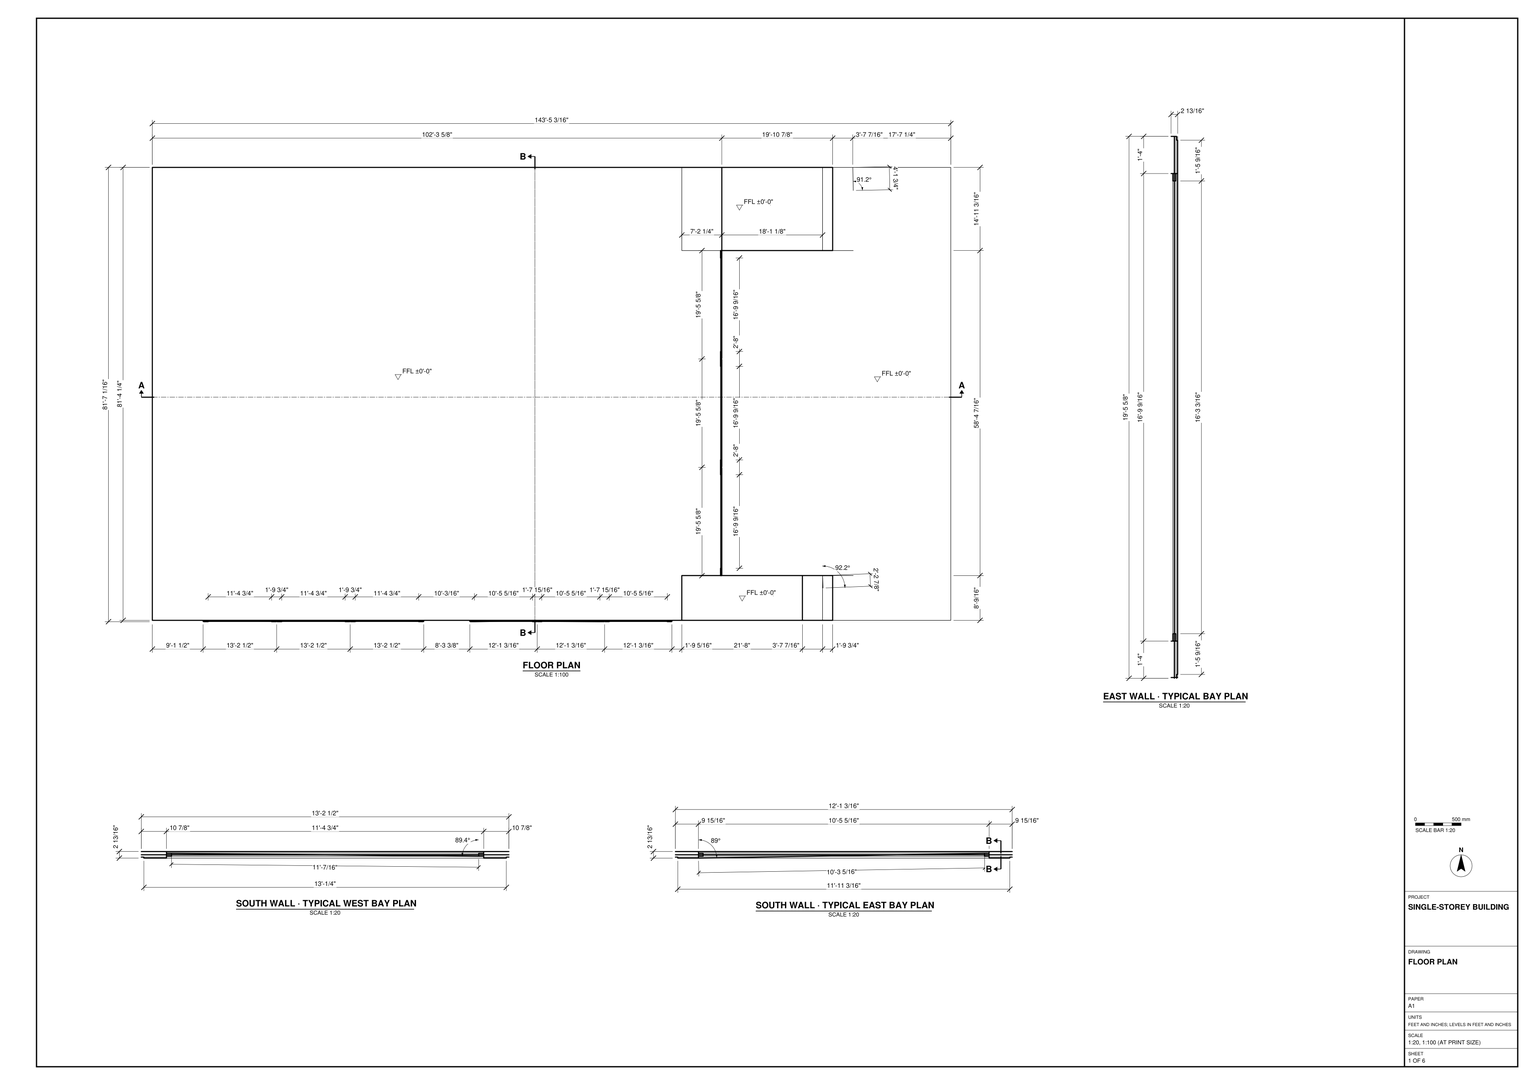
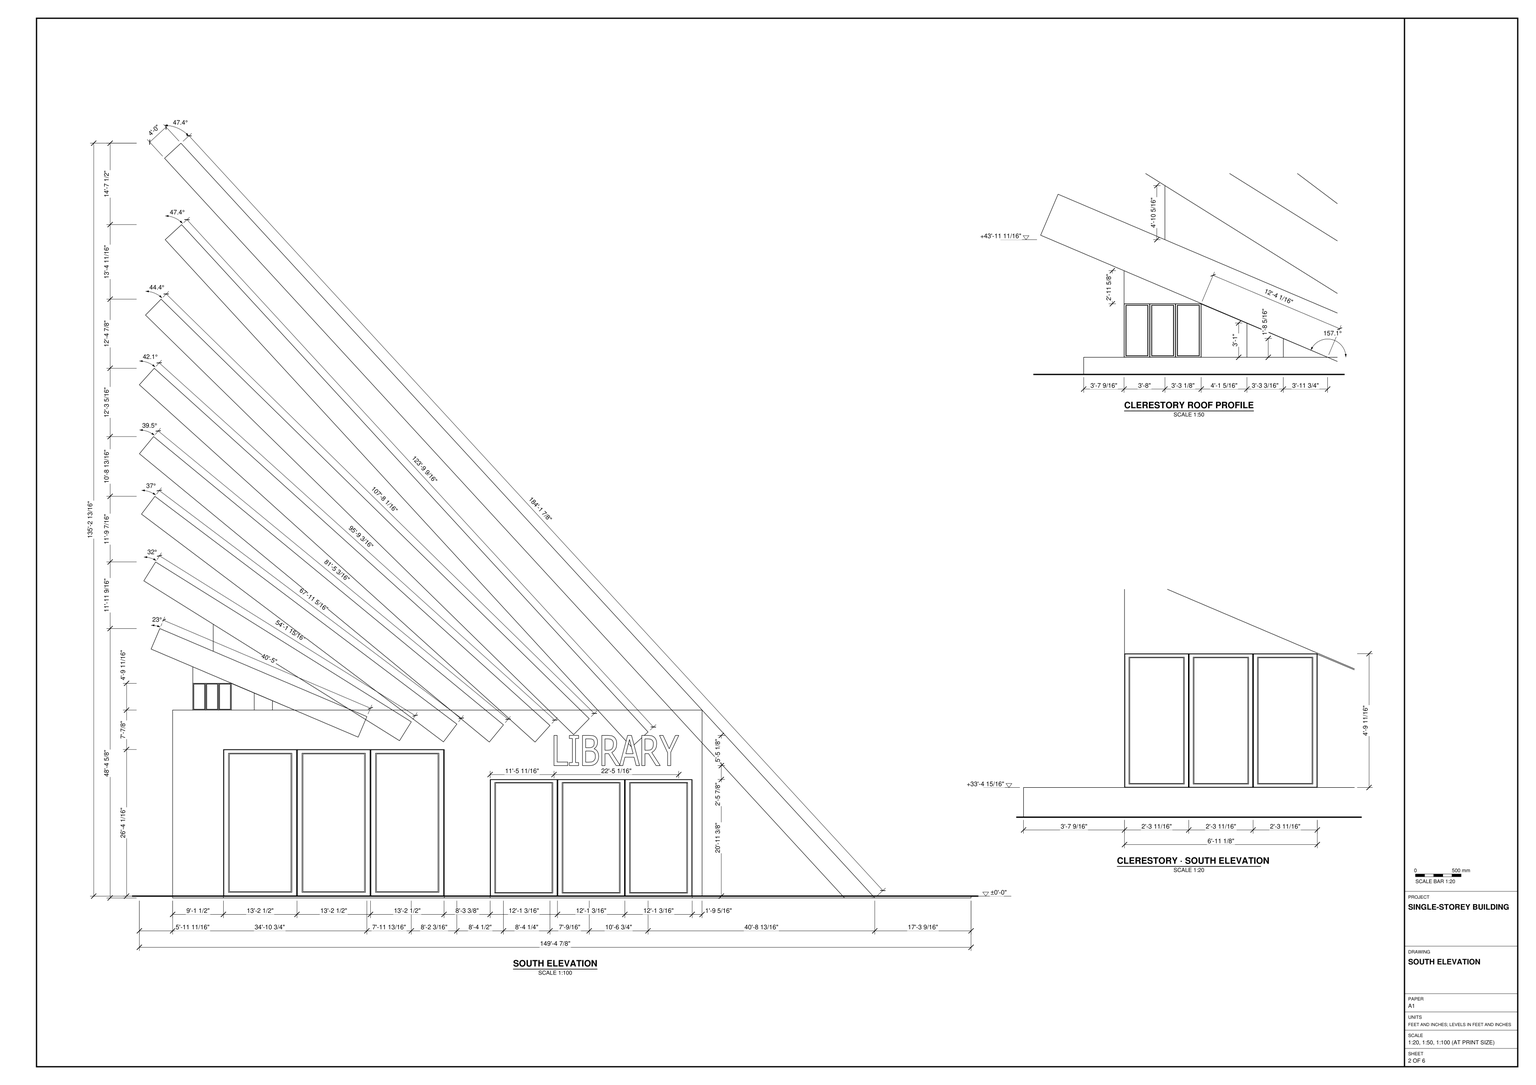
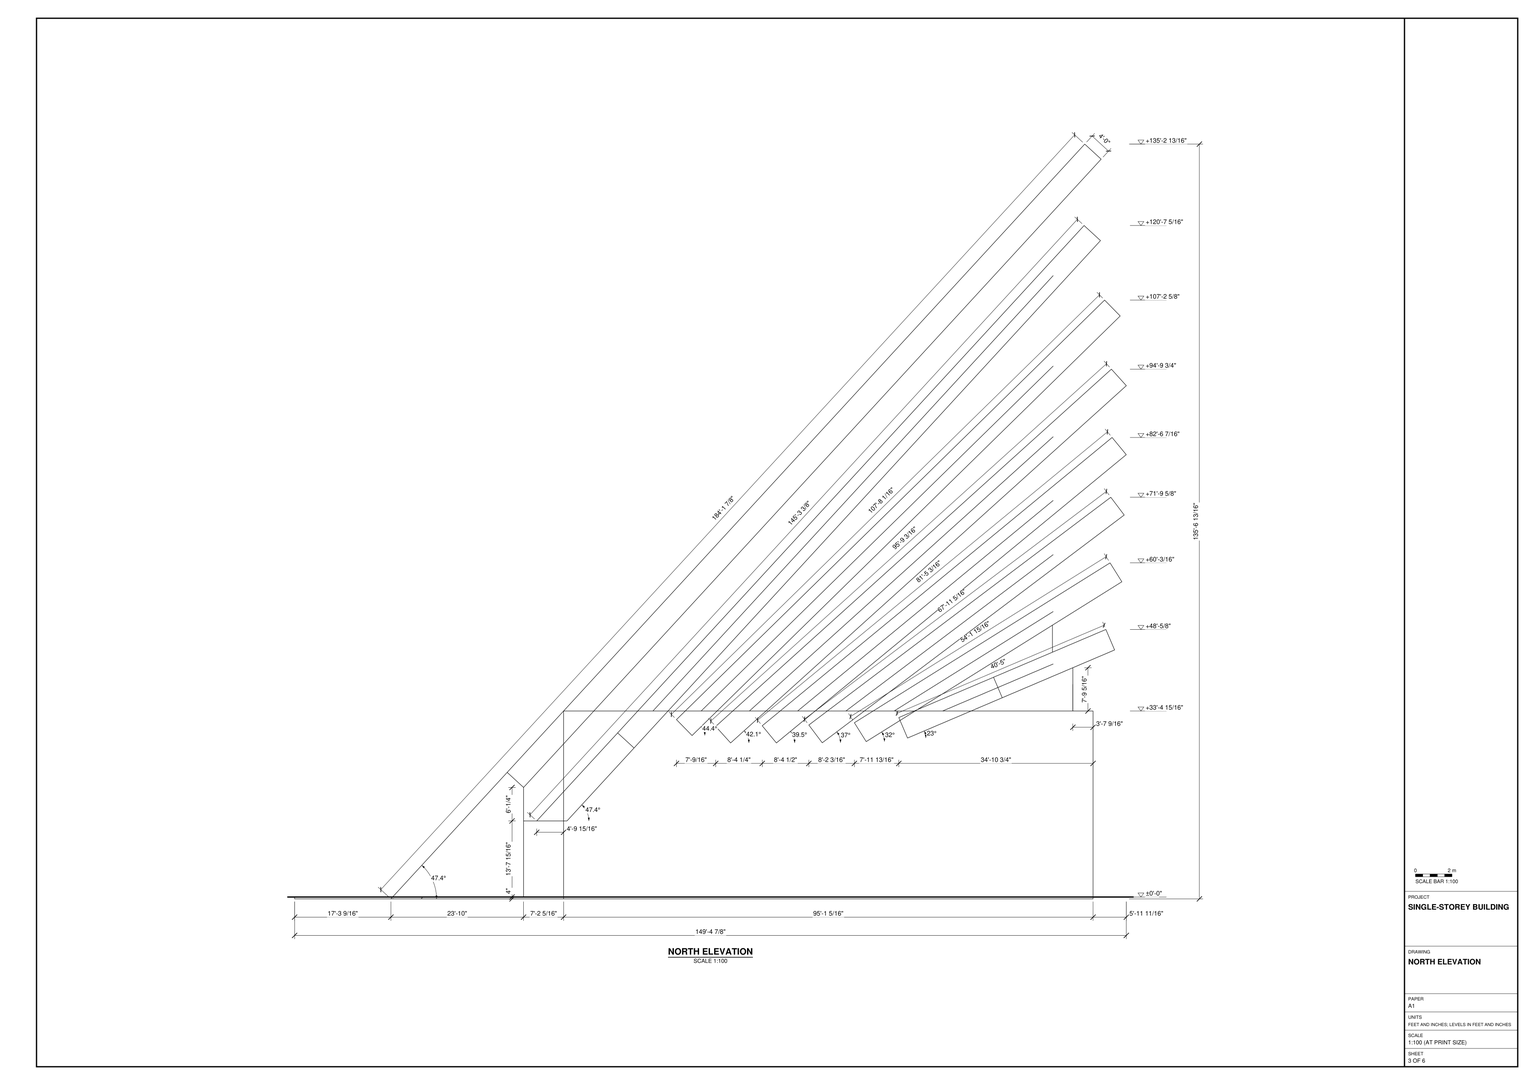
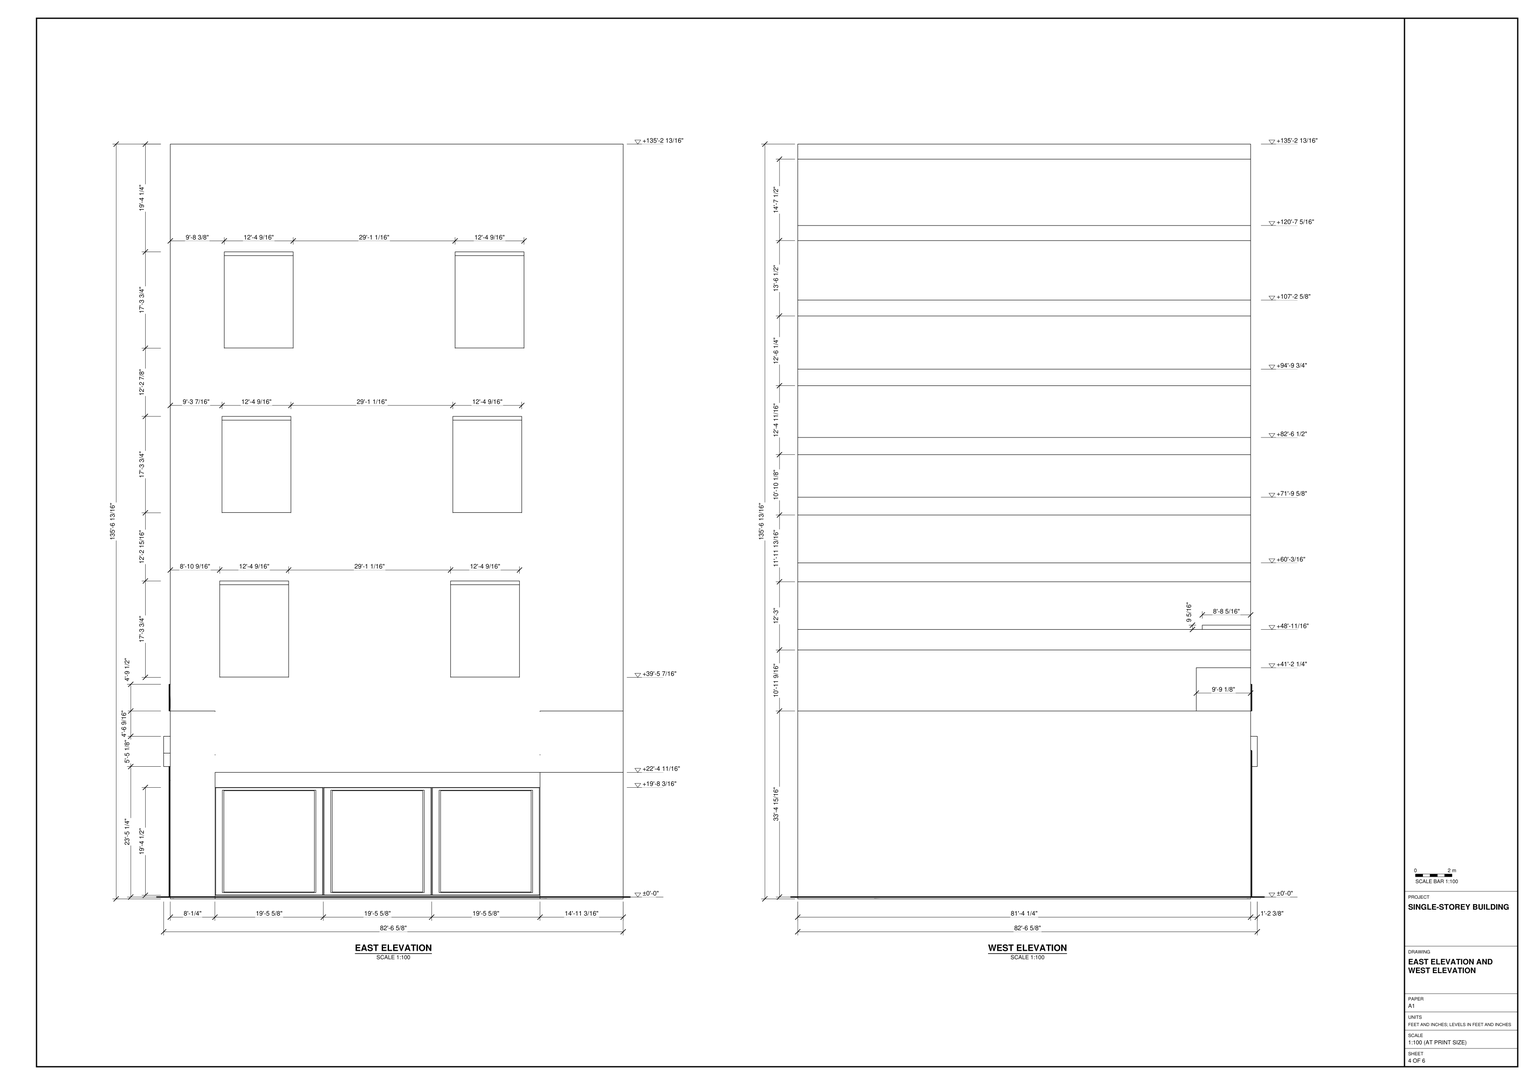
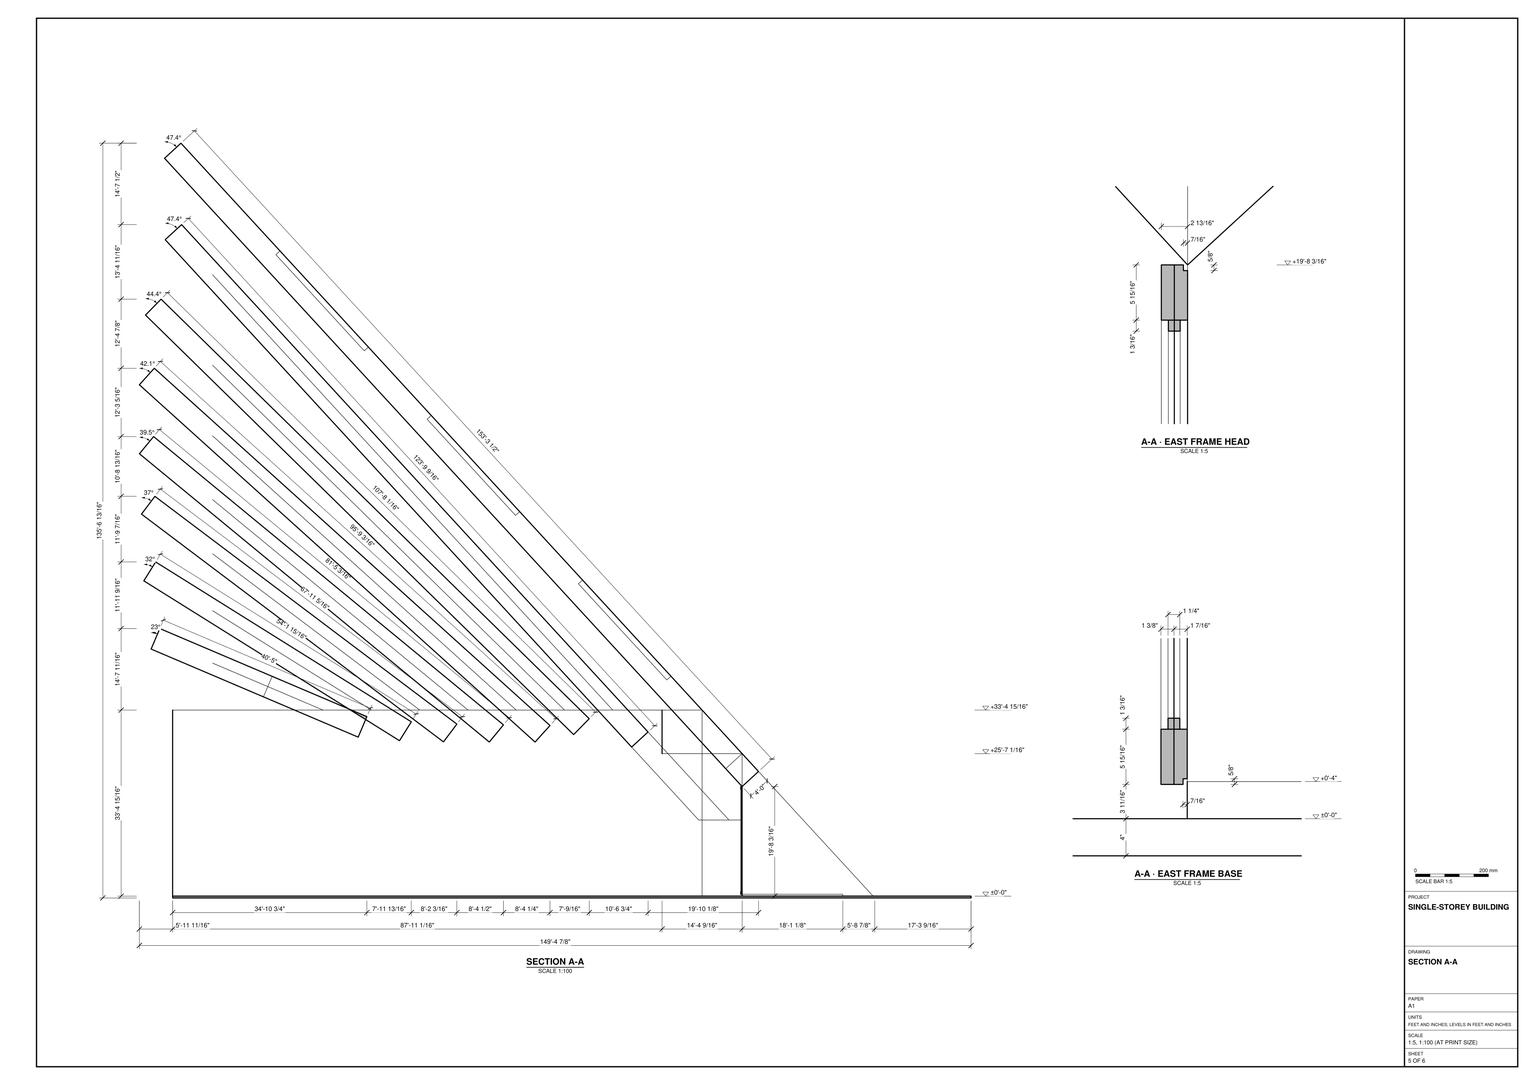
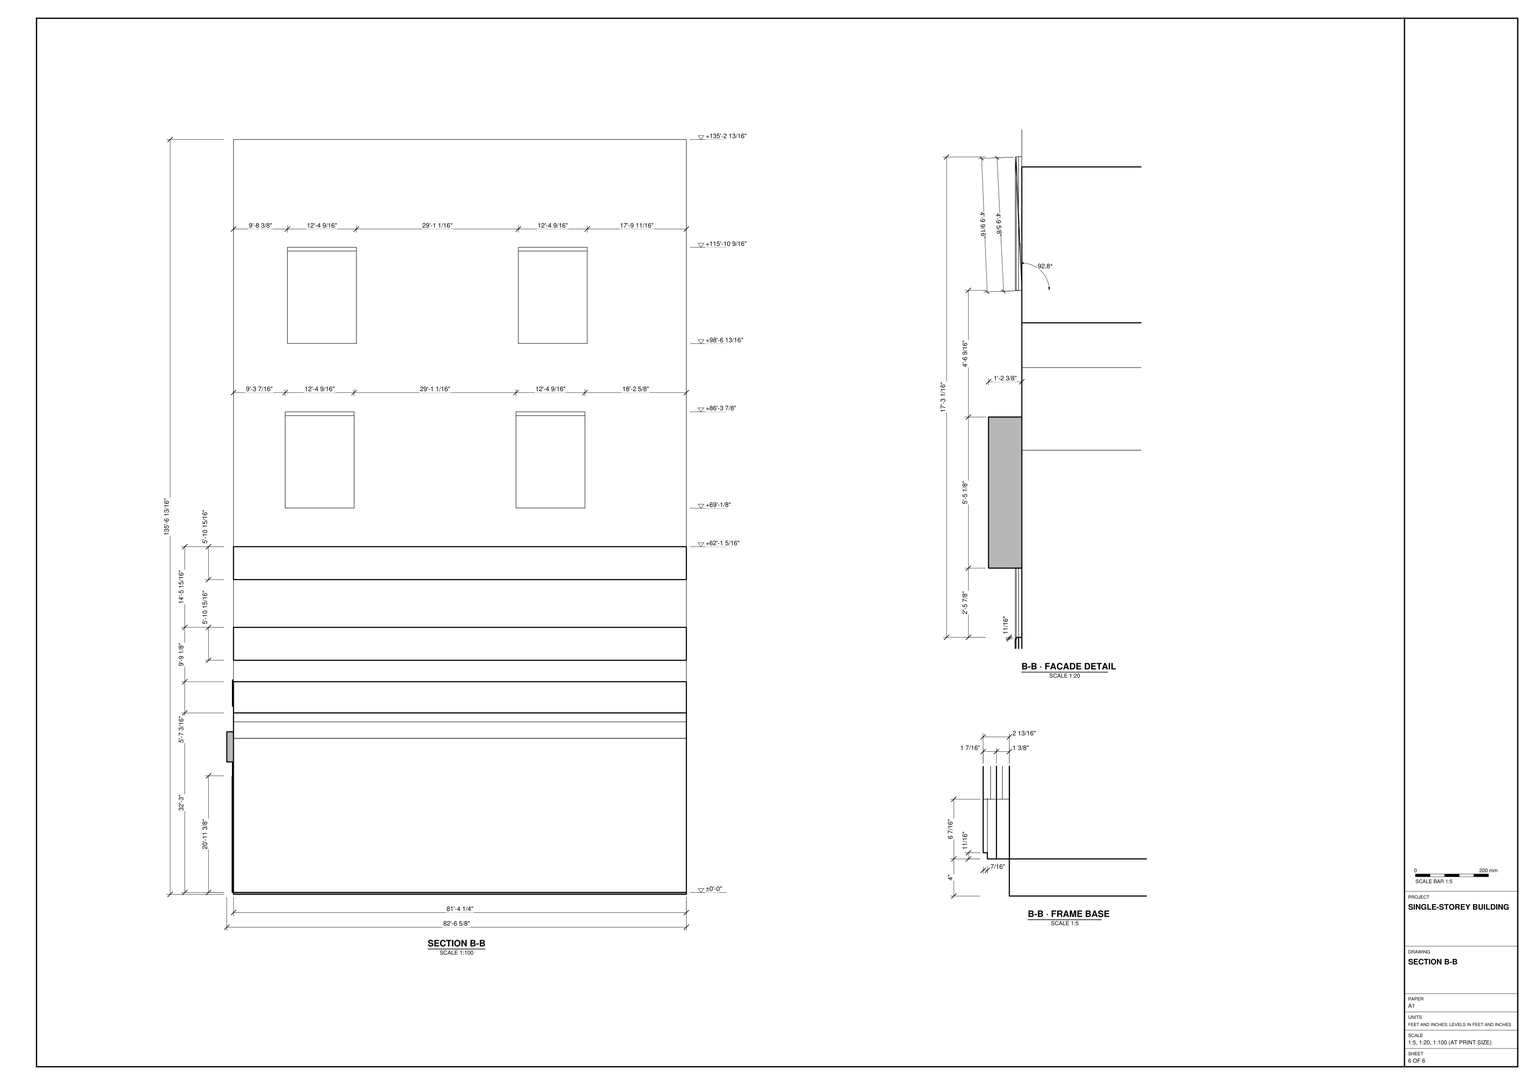
Build the single-storey library in SketchUp from task_files/diagram_01.pdf. Work in feet and inches. The overall model extents are 149'-4 7/8" east to west, 82'-6 5/8" north to south and 135'-6 13/16" vertically. Set the finished ground floor at ±0'-0".

Lay out the slab and walls from the floor plan, including the recessed east wall between the projecting ends. Use the typical bay plans to set the wall and frame thicknesses. On the south wall, form the taller bank of glazed bays to the west and the lower bank to the east, with the library lettering above the lower bank. Keep the broad north wall plain as shown in elevation.

Use the north and south elevations together to set out the inclined roof elements. Give each its drawn thickness, slope and endpoints so that the separate tips form a fan above the building and the longest element reaches the slab to the east. Fit the framed clerestory glazing beneath the lowest inclined element.

Keep walls, slabs, roof elements and any furniture or joinery pieces in separate groups or components, and use components for repeated parts. Decor and loose items may be suitable library components. Save one SketchUp model as output_files/single_storey_library_with_a_fan_shaped_roof.skp.

# SketchUp Ruby script. Lengths in inches.
U = 1.inch
M = Sketchup.active_model
def pt(a) = Geom::Point3d.new(a.map { |v| v * U })
def face(e, loops, mat)
  f = e.add_face(loops[0].map { |a| pt(a) })
  loops[1..].each { |l| e.add_face(l.map { |a| pt(a) }).erase! }
  f.material = f.back_material = mat if mat
  f
end
# faces: each face lists its corners as indices into pts; further lists are holes
def faces(e, pts, list, mat = nil) = list.each { |f| face(e, (f[0].is_a?(Array) ? f : [f]).map { |l| l.map { |i| pts[i] } }, mat) }
# xy, xz, yz: faces in a plane at the given z, y or x. An outline is a flat list of corners, or four numbers for a rectangle; further outlines are holes
def ring(l) = l.size == 4 ? [[l[0], l[1]], [l[2], l[1]], [l[2], l[3]], [l[0], l[3]]] : l.each_slice(2).to_a
def flat(e, list, mat, &to3) = list.each { |f| face(e, (f[0].is_a?(Array) ? f : [f]).map { |l| ring(l).map { |u, v| to3.(u, v) } }, mat) }
def xy(e, z, list, mat = nil) = flat(e, list, mat) { |x, y| [x, y, z] }
def xz(e, y, list, mat = nil) = flat(e, list, mat) { |x, z| [x, y, z] }
def yz(e, x, list, mat = nil) = flat(e, list, mat) { |y, z| [x, y, z] }
def lines(e, pts, list) = list.each { |a, b| e.add_line(pt(pts[a]), pt(pts[b])) }
# prism: a flat outline (further loops are holes) pulled along v
def prism(e, loops, v, mat = nil)
  f = face(e, loops, mat); d = Geom::Vector3d.new(v.map { |x| x * U })
  f.pushpull(f.normal.samedirection?(d) ? d.length : -d.length)
end
def box(e, o, s, mat = nil) = prism(e, [[o, [o[0] + s[0], o[1], o[2]], [o[0] + s[0], o[1] + s[1], o[2]], [o[0], o[1] + s[1], o[2]]]], [0, 0, s[2]], mat)
def at(x, y, z, deg = 0) = Geom::Transformation.translation(pt([x, y, z])) * Geom::Transformation.rotation(ORIGIN, Z_AXIS, deg.degrees)
def axes(o, x, y, z) = Geom::Transformation.new([*x, 0, *y, 0, *z, 0, *pt(o).to_a, 1])
def part(name) = M.definitions.add(name)
# library, detail: a bought-in or finely detailed component or shape, given as its bounding box
def library(name, o, s) = part(name).tap { |d| box(d.entities, o, s) }
def detail(e, o, s) = box(e.add_group.entities, o, s)
def put(e, d, t, mat = nil) = e.add_instance(d, t).tap { |i| i.material = mat if mat }
def group(e, t, mat = nil) = e.add_group.tap { |g| g.transformation = t; g.material = mat if mat }.entities
root = M.entities
M.materials.add("Wine2").color = [0, 0, 0]
M.materials["Wine2"].alpha = 0
M.materials.add("[0130_Gainsboro]").color = [39, 45, 50]
M.materials.add("[Slate]").color = [102, 110, 108]
M.materials.add("[Translucent Glass Safety]").color = [204, 235, 244]
M.materials["[Translucent Glass Safety]"].alpha = 0.5
c1 = part("Framed glazing panel")
xy(c1.entities,0,[[0,-0.98,43.07,0],[0,0,43.07,1.4]],"[0130_Gainsboro]")
xy(c1.entities,0.3,[[0.3,-1.43,42.77,-0.98]],"[0130_Gainsboro]")
xy(c1.entities,2.95,[[2.95,-1.43,40.12,-0.63],[2.95,-0.63,40.12,0],[2.95,0,40.12,0.64],[2.95,0.64,40.12,1.4]],"[0130_Gainsboro]")
xy(c1.entities,3.54,[[3.54,-0.63,39.53,0],[3.54,0,39.53,0.64]],"[0130_Gainsboro]")
xy(c1.entities,111.8125,[[3.54,-0.63,39.53,0],[3.54,0,39.53,0.64]],"[0130_Gainsboro]")
xy(c1.entities,112.4,[[2.95,-1.43,40.12,-0.63],[2.95,-0.63,40.12,0],[2.95,0,40.12,0.64],[2.95,0.64,40.12,1.4]],"[0130_Gainsboro]")
xy(c1.entities,115.05,[[0.3,-1.43,42.77,-0.98]],"[0130_Gainsboro]")
xy(c1.entities,115.35,[[0,-0.98,43.07,0],[0,0,43.07,1.4]],"[0130_Gainsboro]")
xz(c1.entities,-1.43,[[[0.3,0.3,42.77,115.05],[2.95,2.95,40.12,112.4]]],"[0130_Gainsboro]")
xz(c1.entities,-0.98,[[[0,0,43.07,115.35],[0.3,0.3,42.77,115.05]]],"[0130_Gainsboro]")
xz(c1.entities,-0.63,[[[2.95,2.95,40.12,112.4],[3.54,3.54,39.53,111.8125]]],"[0130_Gainsboro]")
xz(c1.entities,0,[[3.54,3.54,39.53,111.8125]],"Wine2")
xz(c1.entities,0,[[[0,0,43.07,115.35],[2.95,2.95,40.12,112.4]],[[2.95,2.95,40.12,112.4],[3.54,3.54,39.53,111.8125]]],"[0130_Gainsboro]")
xz(c1.entities,0.64,[[[2.95,2.95,40.12,112.4],[3.54,3.54,39.53,111.8125]]],"[0130_Gainsboro]")
xz(c1.entities,1.4,[[[0,0,43.07,115.35],[2.95,2.95,40.12,112.4]]],"[0130_Gainsboro]")
yz(c1.entities,0,[[-0.98,0,0,115.35],[0,0,1.4,115.35]],"[0130_Gainsboro]")
yz(c1.entities,0.3,[[-1.43,0.3,-0.98,115.05]],"[0130_Gainsboro]")
yz(c1.entities,2.95,[[-1.43,2.95,-0.63,112.4],[-0.63,2.95,0,112.4],[0,2.95,0.64,112.4],[0.64,2.95,1.4,112.4]],"[0130_Gainsboro]")
yz(c1.entities,3.54,[[-0.63,3.54,0,111.8125],[0,3.54,0.64,111.8125]],"[0130_Gainsboro]")
yz(c1.entities,39.53,[[-0.63,3.54,0,111.8125],[0,3.54,0.64,111.8125]],"[0130_Gainsboro]")
yz(c1.entities,40.12,[[-1.43,2.95,-0.63,112.4],[-0.63,2.95,0,112.4],[0,2.95,0.64,112.4],[0.64,2.95,1.4,112.4]],"[0130_Gainsboro]")
yz(c1.entities,42.77,[[-1.43,0.3,-0.98,115.05]],"[0130_Gainsboro]")
yz(c1.entities,43.07,[[-0.98,0,0,115.35],[0,0,1.4,115.35]],"[0130_Gainsboro]")
c2 = part("Glazed panel assembly")
put(c2.entities,c1,axes([90.57,1.43,0],[1.05148,0,0],[0,1,0],[0,0,1]))
put(c2.entities,c1,axes([0,1.43,0],[1.05148,0,0],[0,1,0],[0,0,1]))
put(c2.entities,c1,axes([45.29,1.43,0],[1.05148,0,0],[0,1,0],[0,0,1]))
c3 = library("LIBRARY",[0.96,0,0],[49.83,9.51,1])
prism(root,[[[936.12,2.83,184.17],[13.24,2.83,1088.42],[13.24,979.08,1088.42],[936.12,979.08,184.17]]],[33.59,0,34.29])
prism(root,[[[852.98,2.83,168.11],[0,2.83,938.18],[0,979.08,938.18],[852.98,979.08,168.11]]],[32.17,0,35.63])
prism(root,[[[754.34,2.83,168.13],[0.15,2.83,789.49],[0.15,979.08,789.49],[754.34,979.08,168.13]]],[30.52,0,37.05])
prism(root,[[[655.5,2.83,168.46],[4.59,2.83,659.39],[4.59,979.08,659.39],[655.5,979.08,168.46]]],[28.9,0,38.32])
xy(root,-167.93,[[71.7,2.83,1792.87,979.08]])
xy(root,-163.93,[[1213.03,2.83,1516.4375,99.4],[1516.4375,2.83,1792.87,2.83,1792.87,979.08,1516.4375,979.08,1516.4375,799.87,1299.3,799.87,1299.3,99.4,1516.4375,99.4],[1299.3,799.87,1516.4375,979.08]])
xy(root,237,[[115.23,2.83,334.62,119.96]])
xz(root,1.43,[[117.51,238.77,140.66,292.91],[145.22,238.77,168.37,292.91],[172.92,238.77,196.08,292.91]])
xz(root,2.83,[[71.7,-167.93,181.19,-163.93],[181.19,-167.93,657.38,152.13],[657.38,-167.93,756.09,-163.93],[756.09,-167.93,1191.71,87.44],[1191.71,-167.93,1520.11,-167.93,1516.4375,-163.93,1191.71,-163.93],
  [1520.11,-167.93,1585.32,-167.93,1581.64,-163.93,1516.4375,-163.93],[1585.32,-167.93,1792.87,-167.93,1792.87,-163.93,1581.64,-163.93],[1516.4375,-163.93,1581.64,-163.93,89.64,1458.875,54.31,1426.39,1213.03,166.08],[1213.03,-163.93,1516.4375,-163.93,1213.03,166.08],[1061.15,157.3125,1096.48,189.8,91.04,1283.4,55.7,1250.91],
  [560.76,171.01,586.21,211.72,35.08,556.26,9.63,515.56,159.23,422.03,450.84,239.73,490.42,222.9,487.76,216.65],[471.64,178.73,487.76,216.65,450.84,239.73,159.23,363.76,44.09,412.73,25.3,368.56,115.23,330.31,334.62,237],[487.76,216.65,490.42,222.9,450.84,239.73]])
xz(root,2.83,[[115.23,237,334.62,237,115.23,330.31],[450.84,239.73,159.23,422.03,159.23,363.76]],"[Translucent Glass Safety]")
xz(root,99.4,[[1585.32,-167.93,1516.4375,-163.93,1516.4375,-159.93,1512.76,-159.93,1299.3,72.24,1334.64,104.72],[1213.03,-163.93,1299.3,-159.93],[1299.3,-163.93,1299.3,-159.93,1512.76,-159.93,1516.4375,-163.93],[1516.4375,-163.93,1512.76,-159.93,1516.4375,-159.93],[1213.03,-159.93,1213.03,143.16,1299.3,143.16,1263.97,110.67,1299.3,72.24,1512.76,-159.93],
  [1299.3,72.24,1263.97,110.67,1299.3,143.16]])
xz(root,107.14,[[450.84,239.73,159.23,422.03,159.23,363.76]])
xz(root,109.39,[[1136.98,301.99,946.5,509.17,955.33,517.29,1145.8125,310.11]])
xz(root,114.29,[[810.9,656.66,620.42,863.84,629.25,871.96,819.73,664.78]])
xz(root,119.18,[[484.82,1011.32,294.33,1218.51,303.17,1226.63,493.65,1019.45]])
xz(root,119.96,[[115.23,237,115.23,330.31,334.62,237]])
xz(root,257.95,[[1136.98,301.99,1145.8125,310.11,955.33,517.29,946.5,509.17]])
xz(root,262.85,[[810.9,656.66,819.73,664.78,629.25,871.96,620.42,863.84]])
xz(root,267.75,[[484.82,1011.32,493.65,1019.45,303.17,1226.63,294.33,1218.51]])
xz(root,607.01,[[1136.98,301.99,946.5,509.17,955.33,517.29,1145.8125,310.11]])
xz(root,611.91,[[810.9,656.66,620.42,863.84,629.25,871.96,819.73,664.78]])
xz(root,616.81,[[484.82,1011.32,294.33,1218.51,303.17,1226.63,493.65,1019.45]])
xz(root,755.58,[[1136.98,301.99,1145.8125,310.11,955.33,517.29,946.5,509.17]])
xz(root,760.47,[[810.9,656.66,819.73,664.78,629.25,871.96,620.42,863.84]])
xz(root,765.37,[[484.82,1011.32,493.65,1019.45,303.17,1226.63,294.33,1218.51]])
xz(root,799.87,[[1520.11,-167.93,1585.32,-167.93,1334.64,104.72,1299.3,72.24,1299.3,-159.93,1516.4375,-159.93,1516.4375,-163.93],[1299.3,-163.93,1516.4375,-159.93],[1299.3,72.24,1299.3,143.16,1263.97,110.67]])
xz(root,979.08,[[71.7,-167.93,1213.03,-163.93],[1213.03,-167.93,1213.03,0,1299.3,0,1299.3,-163.93,1516.4375,-163.93,1520.11,-167.93],[1520.11,-167.93,1516.4375,-163.93,1581.64,-163.93,1585.32,-167.93],[1585.32,-167.93,1581.64,-163.93,1792.87,-163.93,1792.87,-167.93],[1299.3,-163.93,1299.3,72.24,1334.64,104.72,1581.64,-163.93],
  [1205.78,0,1061.15,157.3125,1096.48,189.8,1213.03,63.04,1213.03,0],[1213.03,0,1213.03,63.04,1270.98,0],[1270.98,0,1213.03,63.04,1213.03,166.08,1299.3,72.24,1299.3,0],[1299.3,72.24,1334.64,104.72,89.64,1458.875,54.31,1426.39,1213.03,166.08],[1061.15,157.3125,55.7,1250.91,91.04,1283.4,1096.48,189.8],
  [560.76,171.01,487.76,216.65,490.42,222.9,450.84,239.73,9.63,515.56,35.08,556.26,586.21,211.72],[471.64,178.73,267.46,265.57,286.25,309.74,450.84,239.73,487.76,216.65],[487.76,216.65,450.84,239.73,490.42,222.9],[267.46,265.57,25.3,368.56,44.09,412.73,286.25,309.74]])
yz(root,71.7,[[2.83,-167.93,979.08,-163.93]])
yz(root,115.23,[[2.83,237,119.96,330.31]])
yz(root,159.23,[[2.83,363.76,107.14,422.03]])
yz(root,1126.75,[[99.4,143.16,799.87,237]])
yz(root,1213.03,[[2.83,-163.93,99.4,166.08]])
yz(root,1299.3,[[99.4,-163.93,799.87,-159.93],[799.87,-163.93,979.08,0],[799.87,0,979.08,72.24]])
yz(root,1299.3,[[115.1,-154.29,316.66,66.29],[348.69,-154.29,550.26,66.29],[582.29,-154.29,783.85,66.29]],"[Translucent Glass Safety]")
yz(root,1792.87,[[2.83,-167.93,99.4,-163.93],[99.4,-167.93,799.87,-163.93],[799.87,-167.93,979.08,-163.93]])
p = [[1581.64,2.83,-163.93],[1585.32,2.83,-167.93],[1585.32,99.4,-167.93],[1334.64,99.4,104.72],[1334.64,799.87,104.72],[1334.64,979.08,104.72],
  [89.64,979.08,1458.875],[89.64,2.83,1458.875],[955.33,257.95,517.29],[1145.8125,257.95,310.11],[1145.8125,109.39,310.11],[955.33,109.39,517.29],
  [303.17,765.37,1226.63],[493.65,765.37,1019.45],[493.65,616.81,1019.45],[303.17,616.81,1226.63],[629.25,760.47,871.96],[819.73,760.47,664.78],
  [819.73,611.91,664.78],[629.25,611.91,871.96],[629.25,262.85,871.96],[819.73,262.85,664.78],[819.73,114.29,664.78],[629.25,114.29,871.96],
  [955.33,755.58,517.29],[1145.8125,755.58,310.11],[1145.8125,607.01,310.11],[955.33,607.01,517.29],[303.17,119.18,1226.63],[303.17,267.75,1226.63],
  [493.65,267.75,1019.45],[493.65,119.18,1019.45],[1516.4375,2.83,-163.93],[1516.4375,99.4,-163.93],[1520.11,2.83,-167.93],[1585.32,799.87,-167.93],
  [1581.64,979.08,-163.93],[1299.3,979.08,72.24],[1299.3,799.87,72.24],[1263.97,799.87,110.67],[1263.97,99.4,110.67],[1299.3,99.4,72.24],
  [1512.76,99.4,-159.93],[1213.03,2.83,166.08],[54.31,2.83,1426.39],[54.31,979.08,1426.39],[1213.03,979.08,166.08],[911.25,0.8125,-157.5],
  [911.25,0.8125,81.01],[1036.55,0.01,81.01],[1036.55,0.01,-157.5],[1058.44,2.08,-157.5],[1058.44,2.08,79.73],[1181.76,1.44,79.73],
  [1181.76,1.44,-157.5],[766.04,0.01,-156.22],[766.04,0.01,81.01],[889.36,2.08,81.01],[889.36,2.08,-156.22],[326.67,0.8,-154.23],
  [194.22,2.07,-154.23],[194.22,2.07,142.43],[326.67,0.8,142.43],[352.73,2.07,142.43],[485.17,0.8,142.43],[485.17,0.8,-154.23],
  [352.73,2.07,-154.23],[511.23,2.07,-154.23],[511.23,2.07,142.43],[643.68,0.8,142.43],[643.68,0.8,-154.23],[55.7,979.08,1250.91],
  [1061.15,979.08,157.3125],[1061.15,2.83,157.3125],[55.7,2.83,1250.91],[1096.48,979.08,189.8],[1096.48,2.83,189.8],[487.76,2.83,216.65],
  [487.76,979.08,216.65],[560.76,979.08,171.01],[560.76,2.83,171.01],[586.21,979.08,211.72],[586.21,2.83,211.72],[115.23,2.83,330.31],
  [25.3,2.83,368.56],[25.3,979.08,368.56],[267.46,979.08,265.57],[471.64,979.08,178.73],[471.64,2.83,178.73],[334.62,2.83,237],
  [334.62,119.96,237],[115.23,119.96,330.31],[91.04,979.08,1283.4],[91.04,2.83,1283.4],[35.08,2.83,556.26],[35.08,979.08,556.26],
  [159.23,2.83,422.03],[9.63,2.83,515.56],[9.63,979.08,515.56],[450.84,979.08,239.73],[450.84,2.83,239.73],[450.84,107.14,239.73],
  [159.23,107.14,422.03],[490.42,2.83,222.9],[490.42,979.08,222.9],[44.09,2.83,412.73],[159.23,2.83,363.76],[159.23,107.14,363.76],
  [286.25,979.08,309.74],[44.09,979.08,412.73],[946.5,257.95,509.17],[946.5,109.39,509.17],[1136.98,109.39,301.99],[1136.98,257.95,301.99],
  [946.5,755.58,509.17],[946.5,607.01,509.17],[1136.98,607.01,301.99],[1136.98,755.58,301.99],[620.42,262.85,863.84],[620.42,114.29,863.84],
  [810.9,114.29,656.66],[810.9,262.85,656.66],[620.42,760.47,863.84],[620.42,611.91,863.84],[810.9,611.91,656.66],[810.9,760.47,656.66],
  [294.33,267.75,1218.51],[294.33,119.18,1218.51],[484.82,119.18,1011.32],[484.82,267.75,1011.32],[294.33,765.37,1218.51],[294.33,616.81,1218.51],
  [484.82,616.81,1011.32],[484.82,765.37,1011.32],[1299.3,799.87,143.16],[1126.75,799.87,143.16],[1213.03,99.4,237],[1126.75,99.4,237],
  [1213.03,99.4,143.16],[1126.75,99.4,143.16],[1278.23,99.4,166.08],[1213.03,99.4,166.08],[198.16,2.83,237],[198.16,0.45,294.53],
  [286.875,2.83,237],[286.875,2.13,253.92],[247.65,1.43,270.85],[247.65,2.83,237],[198.16,0,294.53],[286.875,2.13,257.31],
  [247.65,1.43,273.99]]
faces(root,p,[[[0,1,2,3,4,5,6,7],[8,9,10,11],[12,13,14,15],[16,17,18,19],[20,21,22,23],[24,25,26,27],[28,29,30,31]],[32,33,34],[4,35,36,5],[37,38,39,40,41,42,33,32,43,44,45,46],[38,41,40,39],[41,38,4,3],[38,37,5,4],[71,72,73,74],
  [73,72,75,76],[77,78,79,80],[81,82,80,79],[83,84,85,86,87,88,89,90,91],[87,78,77,88],[75,92,93,76],[94,82,81,95],[96,97,98,99,78,77,100,101,102],
  [103,77,78,104],[105,106,107,101,100,103,104,99,108,109],[89,83,91,90],[100,96,102,101],[106,100,101,107],[10,9,113,112],[26,25,117,116],[105,109,85,84],
  [8,11,111,110],[24,27,115,114],[94,95,98,97],[22,21,121,120],[18,17,125,124],[20,23,119,118],[16,19,123,122],[31,30,129,128],
  [14,13,133,132],[29,28,127,126],[12,15,131,130],[71,74,93,92],[6,45,44,7]])
faces(root,p,[[47,48,49,50],[51,52,53,54],[55,56,57,58],[59,60,61,62],[63,64,65,66],[67,68,69,70],[110,111,112,113],[114,115,116,117],
  [118,119,120,121],[122,123,124,125],[126,127,128,129],[130,131,132,133]],"[Translucent Glass Safety]")
lines(root,p,[[134,135],[136,137],[138,139],[140,141],[142,143],[144,145],[146,147],[148,89],[145,149],[146,150]])
put(root,c2,axes([1299.3,99.08,-160.24],[0,5.15812,0],[-1,0,0],[0,0,2.0153]))
put(root,c2,axes([181.19,0,-163.93],[3.5,0,0],[0,1,0],[0,0,2.73993]),"[Translucent Glass Safety]")
put(root,c2,axes([756.09,0.01,-163.93],[3.2064,0,0],[0,1,0],[0,0,2.17916]),"[Translucent Glass Safety]")
put(root,c2,axes([115.23,0,237],[0.6118,0,0],[0,1,0],[0,0,0.5]),"[Translucent Glass Safety]")
put(root,c3,axes([888.55,2.83,117.3],[5.40024,0,0],[0,0,6.85],[0,-14.365,0]),"[Slate]")
g1 = group(root,at(157.76,2.83,0))
xy(g1,-163.93,[[-86.0625,0,1055.26,0,1055.26,96.57,1141.54,96.57,1141.54,797.04,1055.26,797.04,1055.26,976.25,-86.0625,976.25]])
xz(g1,0,[[-86.0625,-163.93,1055.26,237]])
xz(g1,976.25,[[-86.0625,-163.93,1055.26,237]])
yz(g1,-86.0625,[[0,-163.93,976.25,237]])
yz(g1,1055.26,[[0,-163.93,96.57,237]])
p = [[862.72,976.25,237],[0,976.25,1175.36],[446.72,976.25,237],[0,976.25,573.92],[654.72,976.25,237],[0,976.25,828.08],
  [758.72,976.25,237],[0,976.25,980.42],[342.72,976.25,237],[0,976.25,451.26],[238.18,976.25,237],[0,976.25,338.3],
  [550.72,976.25,237],[0,976.25,690.74],[1055.26,976.25,237],[1055.26,797.04,237],[1055.26,797.04,-163.93]]
lines(g1,p,[[0,1],[2,3],[4,5],[6,7],[8,9],[10,11],[12,13],[14,15],[16,15]])
